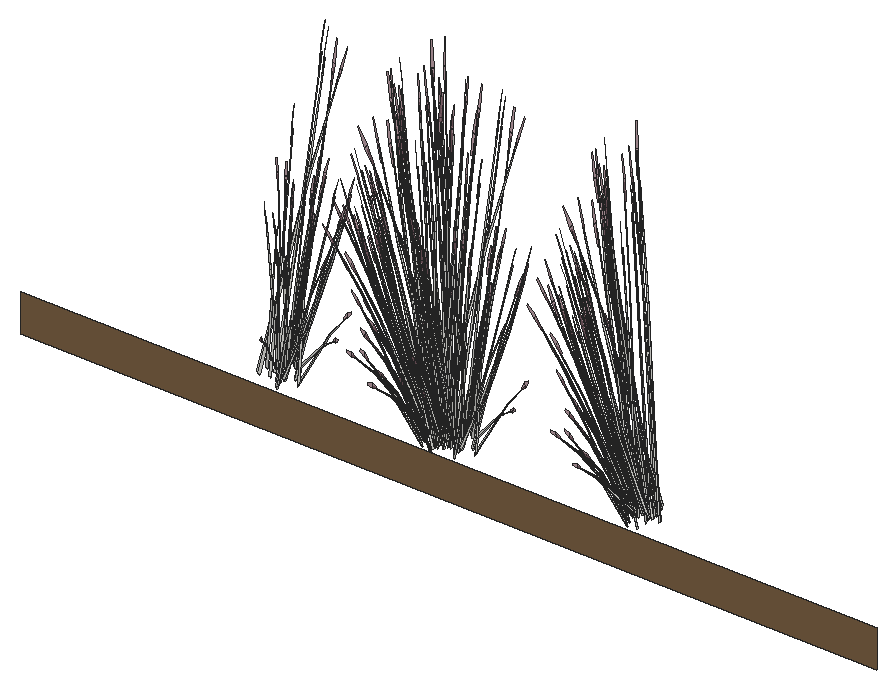
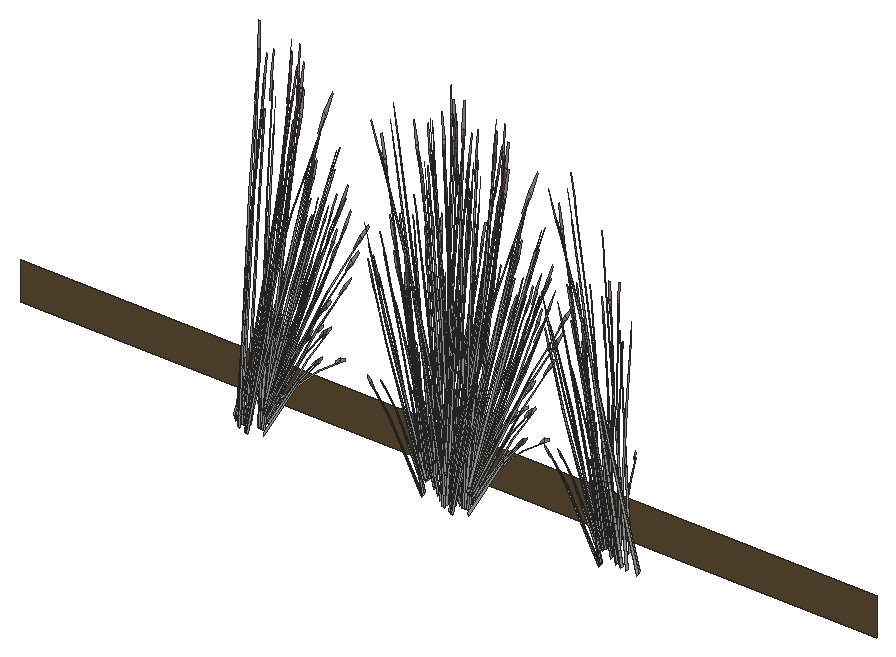
# SketchUp Ruby script. Lengths in inches.
U = 1.inch
M = Sketchup.active_model
def pt(a) = Geom::Point3d.new(a.map { |v| v * U })
def face(e, loops, mat)
  f = e.add_face(loops[0].map { |a| pt(a) })
  loops[1..].each { |l| e.add_face(l.map { |a| pt(a) }).erase! }
  f.material = f.back_material = mat if mat
  f
end
# faces: each face lists its corners as indices into pts; further lists are holes
def faces(e, pts, list, mat = nil) = list.each { |f| face(e, (f[0].is_a?(Array) ? f : [f]).map { |l| l.map { |i| pts[i] } }, mat) }
# xy, xz, yz: faces in a plane at the given z, y or x. An outline is a flat list of corners, or four numbers for a rectangle; further outlines are holes
def ring(l) = l.size == 4 ? [[l[0], l[1]], [l[2], l[1]], [l[2], l[3]], [l[0], l[3]]] : l.each_slice(2).to_a
def flat(e, list, mat, &to3) = list.each { |f| face(e, (f[0].is_a?(Array) ? f : [f]).map { |l| ring(l).map { |u, v| to3.(u, v) } }, mat) }
def xy(e, z, list, mat = nil) = flat(e, list, mat) { |x, y| [x, y, z] }
def xz(e, y, list, mat = nil) = flat(e, list, mat) { |x, z| [x, y, z] }
def yz(e, x, list, mat = nil) = flat(e, list, mat) { |y, z| [x, y, z] }
def lines(e, pts, list) = list.each { |a, b| e.add_line(pt(pts[a]), pt(pts[b])) }
# prism: a flat outline (further loops are holes) pulled along v
def prism(e, loops, v, mat = nil)
  f = face(e, loops, mat); d = Geom::Vector3d.new(v.map { |x| x * U })
  f.pushpull(f.normal.samedirection?(d) ? d.length : -d.length)
end
def box(e, o, s, mat = nil) = prism(e, [[o, [o[0] + s[0], o[1], o[2]], [o[0] + s[0], o[1] + s[1], o[2]], [o[0], o[1] + s[1], o[2]]]], [0, 0, s[2]], mat)
def at(x, y, z, deg = 0) = Geom::Transformation.translation(pt([x, y, z])) * Geom::Transformation.rotation(ORIGIN, Z_AXIS, deg.degrees)
def axes(o, x, y, z) = Geom::Transformation.new([*x, 0, *y, 0, *z, 0, *pt(o).to_a, 1])
def part(name) = M.definitions.add(name)
# library, detail: a bought-in or finely detailed component or shape, given as its bounding box
def library(name, o, s) = part(name).tap { |d| box(d.entities, o, s) }
def detail(e, o, s) = box(e.add_group.entities, o, s)
def put(e, d, t, mat = nil) = e.add_instance(d, t).tap { |i| i.material = mat if mat }
def group(e, t, mat = nil) = e.add_group.tap { |g| g.transformation = t; g.material = mat if mat }.entities
root = M.entities
M.materials.add("LightPink_Translucent").color = [144, 107, 117]
M.materials["LightPink_Translucent"].alpha = 0.75
M.materials.add("Soil_03_1K").color = [122, 96, 67]
c1 = part("blade")
p = [[2.15,0.21,22],[0,0.17,0],[0.09,0.45,0],[2.18,0.31,22],[2.29,0.31,22],[0.38,0.45,0],
  [2.48,0.24,33],[2.49,0.24,33],[2.48,0.22,33]]
faces(c1.entities,p,[[0,1,2,3],[4,5,2,3],[6,3,4,7],[8,0,3,6]])
c2 = part("seeds")
p = [[0.3,-0.1,1.38],[-0.01,-0.03,1.59],[-0.01,-0.03,0.03],[0.14,-0.07,-0.07],[0.29,-0.03,3],[0.15,0.01,3.11]]
faces(c2.entities,p,[[0,1,2,3],[1,0,4,5]],"LightPink_Translucent")
c3 = part("blade with seeds")
put(c3.entities,c1,at(0,0,0))
put(c3.entities,c2,axes([2.4,0.25,30.99],[1.5799,-0.05474,1.17369],[-0.12525,1.92788,0.29478],[-0.07173,-0.02425,1.56792]))
xz(root,2.62,[[45.22,-6,195.77,0.58]],"Soil_03_1K")
put(root,c3,axes([110.6875,10.6,-2.125],[0.17368,0.19618,1.71376],[-0.80256,0.16516,0.13857],[-0.18139,-0.30799,0.73262]))
put(root,c3,axes([146.7,10.6,-2.125],[0.17368,0.19618,1.71376],[-0.80256,0.16516,0.13857],[-0.18139,-0.30799,0.73262]))
put(root,c3,axes([112.01,9.3,-1.28],[-0.11621,-0.08567,1.74944],[-0.77555,0.05431,-0.27667],[-0.12378,-0.20491,0.14031]))
put(root,c3,axes([148.03,9.3,-1.28],[-0.11621,-0.08567,1.74944],[-0.77555,0.05431,-0.27667],[-0.12378,-0.20491,0.14031]))
put(root,c3,axes([113.8125,10.3125,-3.41],[-0.21597,0.12368,1.43002],[-0.64681,-0.21647,-0.30754],[0.1199,-0.26922,0.61141]))
put(root,c3,axes([112.83,10.74,-1.02],[-0.36264,-0.49684,-0.71045],[0.74649,-0.27689,0.08574],[-0.0848,-0.24006,1.00501]))
put(root,c3,axes([148.84,10.74,-1.02],[-0.36264,-0.49684,-0.71045],[0.74649,-0.27689,0.08574],[-0.0848,-0.24006,1.00501]))
put(root,c3,axes([110.47,10.08,-3.41],[-0.04601,0.19989,1.43002],[-0.67263,0.16733,-0.30754],[-0.15723,-0.25836,0.61141]))
put(root,c3,axes([146.48,10.08,-3.41],[-0.04601,0.19989,1.43002],[-0.67263,0.16733,-0.30754],[-0.15723,-0.25836,0.61141]))
put(root,c3,axes([112.2,9.64,-4.51],[-0.12744,0.02202,1.76342],[-0.70477,-0.24781,-0.26939],[0.01183,-0.2067,0.30037]))
put(root,c3,axes([114.34,11.23,-1.02],[0.01977,-0.56521,-0.71045],[0.83252,0.03796,0.08574],[0.08786,-0.23945,1.00501]))
put(root,c3,axes([84.32,10.35,-1.28],[-0.00733,-0.12161,1.74944],[-0.61946,-0.35147,-0.27667],[0.09577,-0.21306,0.14031]))
put(root,c3,axes([115.5,10.35,-1.28],[-0.00733,-0.12161,1.74944],[-0.61946,-0.35147,-0.27667],[0.09577,-0.21306,0.14031]))
put(root,c3,axes([112.9,10.32,-1.47],[0.22906,-0.4699,-0.35414],[0.66828,0.13705,0.4572],[-0.06128,-0.18919,0.87481]))
put(root,c3,axes([82.22,10.94,-2.125],[-0.14147,0.21002,1.71376],[-0.59349,-0.43464,0.13857],[0.26773,-0.27089,0.73262]))
put(root,c3,axes([113.4,10.94,-2.125],[-0.14147,0.21002,1.71376],[-0.59349,-0.43464,0.13857],[0.26773,-0.27089,0.73262]))
put(root,c3,axes([115.33,9.91,-1.29],[-0.07716,0.04667,1.77383],[-0.75601,-0.15746,-0.16761],[-0.02737,-0.20368,0.31391]))
put(root,c3,axes([112.56,10.64,-1.32],[-0.7469,-0.15318,-0.51099],[0.25601,-0.52518,-0.3958],[-0.06849,-0.21144,0.97773]))
put(root,c3,axes([148.57,10.64,-1.32],[-0.7469,-0.15318,-0.51099],[0.25601,-0.52518,-0.3958],[-0.06849,-0.21144,0.97773]))
put(root,c3,axes([113.02,9.33,-3.23],[0.09747,0.35631,1.1486],[-0.54071,-0.19735,0.84392],[0.05818,-0.18244,0.25299]))
put(root,c3,axes([114.17,11.04,-1.32],[-0.54391,-0.41056,-0.51099],[0.57458,-0.35956,-0.3958],[0.08276,-0.2086,0.97773]))
put(root,c3,axes([111.22,9.02,-1.29],[-0.01417,0.07324,1.77383],[-0.6991,0.2658,-0.16761],[-0.20573,-0.13587,0.31391]))
put(root,c3,axes([147.23,9.02,-1.29],[-0.01417,0.07324,1.77383],[-0.6991,0.2658,-0.16761],[-0.20573,-0.13587,0.31391]))
put(root,c3,axes([111.06,10.31,-0.91],[0.84639,-0.15705,0.53763],[0.14689,0.61608,0.4433],[-0.19906,-0.18157,1.11249]))
put(root,c3,axes([147.08,10.31,-0.91],[0.84639,-0.15705,0.53763],[0.14689,0.61608,0.4433],[-0.19906,-0.18157,1.11249]))
put(root,c3,axes([112.98,10.43,-1.27],[0.74868,0.15974,0.48003],[-0.25601,0.52518,0.3958],[-0.04499,-0.20653,0.9933]))
put(root,c3,axes([113.19,10.62,-0.97],[-0.74352,0.28449,-0.1216],[-0.36538,-0.50492,-0.67495],[-0.0981,-0.21277,1.02557]))
put(root,c3,axes([149.21,10.62,-0.97],[-0.74352,0.28449,-0.1216],[-0.36538,-0.50492,-0.67495],[-0.0981,-0.21277,1.02557]))
put(root,c3,axes([114.74,11.26,-0.97],[-0.83505,-0.03027,-0.1216],[0.02282,-0.57322,-0.67495],[0.05801,-0.22077,1.02557]))
put(root,c3,axes([83.5,10.89,-1.47],[0.5141,-0.32171,-0.35414],[0.48666,0.36734,0.4572],[0.07405,-0.18664,0.87481]))
put(root,c3,axes([114.68,10.89,-1.47],[0.5141,-0.32171,-0.35414],[0.48666,0.36734,0.4572],[0.07405,-0.18664,0.87481]))
put(root,c3,axes([110.24,9.76,-3.23],[0.39634,0.21267,1.1486],[-0.57721,0.12784,0.84392],[-0.1235,-0.16344,0.25299]))
put(root,c3,axes([146.25,9.76,-3.23],[0.39634,0.21267,1.1486],[-0.57721,0.12784,0.84392],[-0.1235,-0.16344,0.25299]))
put(root,c3,axes([113.18,10.39,-1.27],[0.55987,-0.20767,0.0643],[0.27403,0.37869,0.50621],[-0.05407,-0.16693,0.77189]))
put(root,c3,axes([111.19,10.88,-1.02],[-0.64788,-0.29534,-0.71045],[0.46044,-0.51755,0.08574],[-0.23473,-0.17635,1.00501]))
put(root,c3,axes([147.21,10.88,-1.02],[-0.64788,-0.29534,-0.71045],[0.46044,-0.51755,0.08574],[-0.23473,-0.17635,1.00501]))
put(root,c3,axes([110.97,10.49,-1.47],[-0.11735,-0.49217,-0.35414],[0.67083,-0.12996,0.4572],[-0.18018,-0.14104,0.87481]))
put(root,c3,axes([146.98,10.49,-1.47],[-0.11735,-0.49217,-0.35414],[0.67083,-0.12996,0.4572],[-0.18018,-0.14104,0.87481]))
put(root,c3,axes([111.26,10.45,-1.27],[0.34533,-0.38816,0.0643],[0.49176,0.22599,0.50621],[-0.15898,-0.12445,0.77189]))
put(root,c3,axes([147.27,10.45,-1.27],[0.34533,-0.38816,0.0643],[0.49176,0.22599,0.50621],[-0.15898,-0.12445,0.77189]))
put(root,c3,axes([109.92,10.4,-4.51],[-0.0736,0.08049,1.76342],[-0.74378,0.17355,-0.26939],[-0.17968,-0.15788,0.30037]))
put(root,c3,axes([145.9375,10.4,-4.51],[-0.0736,0.08049,1.76342],[-0.74378,0.17355,-0.26939],[-0.17968,-0.15788,0.30037]))
put(root,c3,axes([111.15,12.61,-3.9],[-0.31203,-0.62659,-0.69835],[0.89884,-0.22566,-0.18329],[-0.03449,-0.21218,1.54149]))
put(root,c3,axes([147.16,12.61,-3.9],[-0.31203,-0.62659,-0.69835],[0.89884,-0.22566,-0.18329],[-0.03449,-0.21218,1.54149]))
put(root,c3,axes([109.53,11.21,-2.125],[0.28223,0.10528,1.71376],[-0.58406,0.44165,0.13857],[-0.36402,-0.19924,0.73262]))
put(root,c3,axes([145.54,11.21,-2.125],[0.28223,0.10528,1.71376],[-0.58406,0.44165,0.13857],[-0.36402,-0.19924,0.73262]))
put(root,c3,axes([84.15,10.69,-4.51],[-0.11372,-0.04814,1.76342],[-0.29211,-0.53779,-0.26939],[0.19706,-0.14594,0.30037]))
put(root,c3,axes([115.32,10.69,-4.51],[-0.11372,-0.04814,1.76342],[-0.29211,-0.53779,-0.26939],[0.19706,-0.14594,0.30037]))
put(root,c3,axes([112.97,10.82,-0.95],[-0.22906,0.4699,0.35414],[-0.66828,-0.13705,-0.4572],[-0.06128,-0.18919,0.87481]))
put(root,c3,axes([148.98,10.82,-0.95],[-0.22906,0.4699,0.35414],[-0.66828,-0.13705,-0.4572],[-0.06128,-0.18919,0.87481]))
put(root,c3,axes([110.89,10.9,-1.32],[-0.74975,0.14525,-0.51099],[-0.13115,-0.55007,-0.3958],[-0.20138,-0.15763,0.97773]))
put(root,c3,axes([146.9,10.9,-1.32],[-0.74975,0.14525,-0.51099],[-0.13115,-0.55007,-0.3958],[-0.20138,-0.15763,0.97773]))
put(root,c3,axes([83.5,11.01,-1.27],[0.54105,0.41691,0.48003],[-0.57458,0.35956,0.3958],[0.0998,-0.1956,0.9933]))
put(root,c3,axes([114.68,11.01,-1.27],[0.54105,0.41691,0.48003],[-0.57458,0.35956,0.3958],[0.0998,-0.1956,0.9933]))
put(root,c3,axes([111.41,10.41,-0.57],[-0.50709,0.58578,-0.13619],[-0.73436,-0.33748,-0.75594],[-0.25527,-0.1655,1.14864]))
put(root,c3,axes([147.43,10.41,-0.57],[-0.50709,0.58578,-0.13619],[-0.73436,-0.33748,-0.75594],[-0.25527,-0.1655,1.14864]))
put(root,c3,axes([83.7,11.05,-1.27],[0.62439,0.02847,0.0643],[-0.01712,0.42991,0.50621],[0.06534,-0.16468,0.77189]))
put(root,c3,axes([114.88,11.05,-1.27],[0.62439,0.02847,0.0643],[-0.01712,0.42991,0.50621],[0.06534,-0.16468,0.77189]))
put(root,c3,axes([114.41,11.35,-0.95],[-0.5141,0.32171,0.35414],[-0.48666,-0.36734,-0.4572],[0.07405,-0.18664,0.87481]))
put(root,c3,axes([84.14,12.21,-1.02],[0.39688,-0.48213,-0.71045],[0.69548,0.34264,0.08574],[0.23697,-0.17468,1.00501]))
put(root,c3,axes([115.32,12.21,-1.02],[0.39688,-0.48213,-0.71045],[0.69548,0.34264,0.08574],[0.23697,-0.17468,1.00501]))
put(root,c3,axes([111.03,10.81,-3.625],[-0.47504,-0.61229,0],[0.79476,-0.34146,-0.51607],[0.18101,-0.07777,1.63711]))
put(root,c3,axes([84.12,11.99,-1.32],[-0.19519,-0.55794,-0.51099],[0.73919,-0.0976,-0.3958],[0.21183,-0.14986,0.97773]))
put(root,c3,axes([115.3,11.99,-1.32],[-0.19519,-0.55794,-0.51099],[0.73919,-0.0976,-0.3958],[0.21183,-0.14986,0.97773]))
put(root,c3,axes([112.07,10.07,-3.87],[-0.52505,0.35054,-0.03893],[-0.48109,-0.38392,-0.17649],[-0.03387,-0.10878,0.58215]))
put(root,c3,axes([148.08,10.07,-3.87],[-0.52505,0.35054,-0.03893],[-0.48109,-0.38392,-0.17649],[-0.03387,-0.10878,0.58215]))
put(root,c3,axes([109.47,10.24,-1.28],[-0.16348,-0.00431,1.74944],[-0.52047,0.43131,-0.27667],[-0.2777,-0.08813,0.14031]))
put(root,c3,axes([145.48,10.24,-1.28],[-0.16348,-0.00431,1.74944],[-0.52047,0.43131,-0.27667],[-0.2777,-0.08813,0.14031]))
put(root,c3,axes([84.47,12.39,-0.97],[-0.70283,-0.33692,-0.1216],[0.40491,-0.48793,-0.67495],[0.19857,-0.16961,1.02557]))
put(root,c3,axes([115.65,12.39,-0.97],[-0.70283,-0.33692,-0.1216],[0.40491,-0.48793,-0.67495],[0.19857,-0.16961,1.02557]))
put(root,c3,axes([112.74,14.22,-2.67],[0.65659,0.2464,1.51261],[-0.64324,0.53082,0.59816],[-0.28812,-0.31461,1.26806]))
put(root,c3,axes([148.76,14.22,-2.67],[0.65659,0.2464,1.51261],[-0.64324,0.53082,0.59816],[-0.28812,-0.31461,1.26806]))
put(root,c3,axes([111.37,10.89,-0.95],[0.11735,0.49217,0.35414],[-0.67083,0.12996,-0.4572],[-0.18018,-0.14104,0.87481]))
put(root,c3,axes([147.38,10.89,-0.95],[0.11735,0.49217,0.35414],[-0.67083,0.12996,-0.4572],[-0.18018,-0.14104,0.87481]))
put(root,c3,axes([109.3125,12.52,-3.98],[0,-0.61104,-0.49651],[0.85008,0,0],[0,-0.13917,1.57504]))
put(root,c3,axes([145.32,12.52,-3.98],[0,-0.61104,-0.49651],[0.85008,0,0],[0,-0.13917,1.57504]))
put(root,c3,axes([111.67,10.71,-3.98],[0.7111,-0.30552,-0.49651],[0.42504,0.54784,0],[0.16196,-0.06958,1.57504]))
put(root,c3,axes([84.72,11.77,-3.41],[-0.27143,-0.0181,1.43002],[-0.27808,-0.48551,-0.30754],[0.33346,-0.13735,0.61141]))
put(root,c3,axes([115.89,11.77,-3.41],[-0.27143,-0.0181,1.43002],[-0.27808,-0.48551,-0.30754],[0.33346,-0.13735,0.61141]))
put(root,c3,axes([109.35,11.21,-0.91],[0.62747,-0.45094,0.53763],[0.54116,0.47889,0.4433],[-0.29439,-0.08318,1.11249]))
put(root,c3,axes([145.36,11.21,-0.91],[0.62747,-0.45094,0.53763],[0.54116,0.47889,0.4433],[-0.29439,-0.08318,1.11249]))
put(root,c3,axes([86.2,12.24,-1.29],[-0.09924,-0.00464,1.77383],[-0.4121,-0.49725,-0.16761],[0.1655,-0.1635,0.31391]))
put(root,c3,axes([117.38,12.24,-1.29],[-0.09924,-0.00464,1.77383],[-0.4121,-0.49725,-0.16761],[0.1655,-0.1635,0.31391]))
put(root,c3,axes([81.34,11.97,-3.94],[0.51177,-0.45928,-0.62353],[0.63575,0.41646,-0.16365],[0.20507,-0.11457,1.37633]))
put(root,c3,axes([112.52,11.97,-3.94],[0.51177,-0.45928,-0.62353],[0.63575,0.41646,-0.16365],[0.20507,-0.11457,1.37633]))
put(root,c3,axes([85.03,10.875,-3.23],[-0.25308,0.31105,1.1486],[-0.21753,-0.4179,0.84392],[0.20902,-0.10472,0.25299]))
put(root,c3,axes([116.21,10.875,-3.23],[-0.25308,0.31105,1.1486],[-0.21753,-0.4179,0.84392],[0.20902,-0.10472,0.25299]))
put(root,c3,axes([84.67,12.04,-1.47],[0.66138,-0.08733,-0.35414],[0.17464,0.49921,0.4572],[0.18953,-0.13408,0.87481]))
put(root,c3,axes([115.84,12.04,-1.47],[0.66138,-0.08733,-0.35414],[0.17464,0.49921,0.4572],[0.18953,-0.13408,0.87481]))
put(root,c3,axes([109.64,11.21,-1.27],[0.03826,-0.46465,0.0643],[0.57772,0.01274,0.50621],[-0.2213,-0.04862,0.77189]))
put(root,c3,axes([145.65,11.21,-1.27],[0.03826,-0.46465,0.0643],[0.57772,0.01274,0.50621],[-0.2213,-0.04862,0.77189]))
put(root,c3,axes([111.625,12.77,-3.79],[0.36864,-0.55059,-0.44739],[0.76598,0.26498,0.21531],[0,-0.12692,1.43643]))
put(root,c3,axes([109.42,11.36,-1.47],[-0.43232,-0.38257,-0.35414],[0.49364,-0.36215,0.4572],[-0.25081,-0.0551,0.87481]))
put(root,c3,axes([145.43,11.36,-1.47],[-0.43232,-0.38257,-0.35414],[0.49364,-0.36215,0.4572],[-0.25081,-0.0551,0.87481]))
put(root,c3,axes([111.96,12.5,-3.33],[-0.08854,-0.69723,-0.29095],[0.92215,-0.04216,-0.50002],[0.16238,-0.09287,1.59708]))
put(root,c3,axes([109.68,12.54,-3.97],[0.53038,-0.38124,-0.30978],[0.53038,0.38124,0.30978],[0,-0.1228,1.38974]))
put(root,c3,axes([145.6875,12.54,-3.97],[0.53038,-0.38124,-0.30978],[0.53038,0.38124,0.30978],[0,-0.1228,1.38974]))
put(root,c3,axes([109.46,10.71,-3.87],[-0.21918,0.49894,-0.03893],[-0.6746,-0.15348,-0.17649],[-0.10242,-0.08161,0.58215]))
put(root,c3,axes([145.47,10.71,-3.87],[-0.21918,0.49894,-0.03893],[-0.6746,-0.15348,-0.17649],[-0.10242,-0.08161,0.58215]))
put(root,c3,axes([84.13,12.34,-0.95],[-0.66138,0.08733,0.35414],[-0.17464,-0.49921,-0.4572],[0.18953,-0.13408,0.87481]))
put(root,c3,axes([115.3,12.34,-0.95],[-0.66138,0.08733,0.35414],[-0.17464,-0.49921,-0.4572],[0.18953,-0.13408,0.87481]))
put(root,c3,axes([111.53,13.23,-3.33],[-0.85568,-0.29155,-0.29095],[0.41201,-0.61537,-0.50002],[-0.02689,-0.15109,1.59708]))
put(root,c3,axes([147.55,13.23,-3.33],[-0.85568,-0.29155,-0.29095],[0.41201,-0.61537,-0.50002],[-0.02689,-0.15109,1.59708]))
put(root,c3,axes([109.1,12.99,-3.625],[-0.95008,0,0],[0,-0.68292,-0.51607],[0,-0.15554,1.63711]))
put(root,c3,axes([145.11,12.99,-3.625],[-0.95008,0,0],[0,-0.68292,-0.51607],[0,-0.15554,1.63711]))
put(root,c3,axes([109.26,11.76,-3.41],[0.14835,0.17012,1.43002],[-0.34183,0.46242,-0.30754],[-0.351,-0.11053,0.61141]))
put(root,c3,axes([145.27,11.76,-3.41],[0.14835,0.17012,1.43002],[-0.34183,0.46242,-0.30754],[-0.351,-0.11053,0.61141]))
put(root,c3,axes([111.84,10.95,-3.97],[0.70886,0.15119,-0.30978],[-0.17848,0.53243,0.30978],[0.1429,-0.0614,1.38974]))
put(root,c3,axes([109.875,11.61,-1.02],[-0.75952,-0.01471,-0.71045],[0.05101,-0.61953,0.08574],[-0.32177,-0.06538,1.00501]))
put(root,c3,axes([145.89,11.61,-1.02],[-0.75952,-0.01471,-0.71045],[0.05101,-0.61953,0.08574],[-0.32177,-0.06538,1.00501]))
put(root,c3,axes([84.73,12.26,-1.27],[0.52161,0.25698,0.0643],[-0.30368,0.36595,0.50621],[0.16723,-0.11831,0.77189]))
put(root,c3,axes([115.9,12.26,-1.27],[0.52161,0.25698,0.0643],[-0.30368,0.36595,0.50621],[0.16723,-0.11831,0.77189]))
put(root,c3,axes([84.58,12.15,-1.27],[0.18844,0.56237,0.48003],[-0.73919,0.0976,0.3958],[0.21785,-0.13226,0.9933]))
put(root,c3,axes([115.76,12.15,-1.27],[0.18844,0.56237,0.48003],[-0.73919,0.0976,0.3958],[0.21785,-0.13226,0.9933]))
put(root,c3,axes([86.58,12.83,-1.28],[0.10543,-0.09307,1.74944],[-0.13495,-0.57092,-0.27667],[0.26455,-0.10825,0.14031]))
put(root,c3,axes([117.75,12.83,-1.28],[0.10543,-0.09307,1.74944],[-0.13495,-0.57092,-0.27667],[0.26455,-0.10825,0.14031]))
put(root,c3,axes([109.83,12.81,-3.67],[-0.70674,0.51372,0.30756],[-0.70717,-0.50832,-0.36492],[-0.02468,-0.14589,1.64885]))
put(root,c3,axes([145.85,12.81,-3.67],[-0.70674,0.51372,0.30756],[-0.70717,-0.50832,-0.36492],[-0.02468,-0.14589,1.64885]))
put(root,c3,axes([108.84,10.6,-1.29],[0.05633,0.06098,1.77383],[-0.27155,0.54815,-0.16761],[-0.27501,0.00397,0.31391]))
put(root,c3,axes([144.86,10.6,-1.29],[0.05633,0.06098,1.77383],[-0.27155,0.54815,-0.16761],[-0.27501,0.00397,0.31391]))
put(root,c3,axes([112.08,13.04,-3.57],[0.8561,0.29616,0.24065],[-0.41201,0.61537,0.50002],[0,-0.14185,1.60543]))
put(root,c3,axes([111.75,13.875,-3.5625],[0.20138,-0.72405,-0.23429],[0.95485,0.12621,0.51271],[-0.16685,-0.09999,1.5644]))
put(root,c3,axes([147.76,13.875,-3.5625],[0.20138,-0.72405,-0.23429],[0.95485,0.12621,0.51271],[-0.16685,-0.09999,1.5644]))
put(root,c3,axes([109.62,11.74,-1.32],[-0.55171,0.40476,-0.51099],[-0.48318,-0.42758,-0.3958],[-0.28031,-0.06159,0.97773]))
put(root,c3,axes([145.63,11.74,-1.32],[-0.55171,0.40476,-0.51099],[-0.48318,-0.42758,-0.3958],[-0.28031,-0.06159,0.97773]))
put(root,c3,axes([110.03,11.56,-0.95],[0.43232,0.38257,0.35414],[-0.49364,0.36215,-0.4572],[-0.25081,-0.0551,0.87481]))
put(root,c3,axes([146.04,11.56,-0.95],[0.43232,0.38257,0.35414],[-0.49364,0.36215,-0.4572],[-0.25081,-0.0551,0.87481]))
put(root,c3,axes([108.38,12.28,-3.23],[0.48508,-0.04372,1.1486],[-0.3077,0.38525,0.84392],[-0.23971,-0.05779,0.25299]))
put(root,c3,axes([144.39,12.28,-3.23],[0.48508,-0.04372,1.1486],[-0.3077,0.38525,0.84392],[-0.23971,-0.05779,0.25299]))
put(root,c3,axes([111.81,12.63,-3.28],[-0.82508,0.03772,0.44739],[-0.07462,-0.62614,-0.21531],[0.14771,-0.06346,1.43643]))
put(root,c3,axes([109.91,11.32,-0.97],[-0.04068,0.62141,-0.1216],[-0.77029,-0.01698,-0.67495],[-0.29667,-0.04317,1.02557]))
put(root,c3,axes([145.92,11.32,-0.97],[-0.04068,0.62141,-0.1216],[-0.77029,-0.01698,-0.67495],[-0.29667,-0.04317,1.02557]))
put(root,c3,axes([109.68,13.09,-3.52],[0,0.61104,0.49651],[-0.85008,0,0],[0,-0.13917,1.57504]))
put(root,c3,axes([145.6875,13.09,-3.52],[0,0.61104,0.49651],[-0.85008,0,0],[0,-0.13917,1.57504]))
put(root,c3,axes([84.5,13.7,-0.97],[-0.38229,-0.5533,-0.1216],[0.6785,-0.2719,-0.67495],[0.28593,-0.073,1.02557]))
put(root,c3,axes([115.68,13.7,-0.97],[-0.38229,-0.5533,-0.1216],[0.6785,-0.2719,-0.67495],[0.28593,-0.073,1.02557]))
put(root,c3,axes([84.47,13.22,-1.32],[0.20584,-0.55581,-0.51099],[0.70573,0.19051,-0.3958],[0.28414,-0.05097,0.97773]))
put(root,c3,axes([115.64,13.22,-1.32],[0.20584,-0.55581,-0.51099],[0.70573,0.19051,-0.3958],[0.28414,-0.05097,0.97773]))
put(root,c3,axes([83.35,10.96,-3.625],[0.47504,-0.61229,0],[0.79476,0.34146,-0.51607],[0.18101,0.07777,1.63711]))
put(root,c3,axes([114.53,10.96,-3.625],[0.47504,-0.61229,0],[0.79476,0.34146,-0.51607],[0.18101,0.07777,1.63711]))
put(root,c3,axes([108.93,12.17,-2.125],[0.31515,-0.01384,1.71376],[-0.20907,0.5998,0.13857],[-0.44912,-0.0371,0.73262]))
put(root,c3,axes([144.94,12.17,-2.125],[0.31515,-0.01384,1.71376],[-0.20907,0.5998,0.13857],[-0.44912,-0.0371,0.73262]))
put(root,c3,axes([111.68,13.58,-3.79],[-0.45644,-0.51287,-0.44739],[0.69137,-0.36116,0.21531],[-0.14771,-0.06346,1.43643]))
put(root,c3,axes([147.7,13.58,-3.79],[-0.45644,-0.51287,-0.44739],[0.69137,-0.36116,0.21531],[-0.14771,-0.06346,1.43643]))
put(root,c3,axes([111.78,12.86,-3.64],[0.33034,0.68327,0.45755],[-0.94388,0.2376,0.17955],[0.01154,-0.12555,1.58856]))
put(root,c3,axes([85.22,13.38,-4.02],[-0.48937,0.07333,1.41583],[-0.07789,-0.58369,0.08104],[0.34275,-0.08835,0.80566]))
put(root,c3,axes([116.4,13.38,-4.02],[-0.48937,0.07333,1.41583],[-0.07789,-0.58369,0.08104],[0.34275,-0.08835,0.80566]))
put(root,c3,axes([86.11,12.86,-3.74],[-0.47106,-0.39072,-0.06488],[0.51591,-0.35801,-0.29416],[0.14618,-0.02521,0.97024]))
put(root,c3,axes([117.29,12.86,-3.74],[-0.47106,-0.39072,-0.06488],[0.51591,-0.35801,-0.29416],[0.14618,-0.02521,0.97024]))
put(root,c3,axes([111.61,13.4,-3.28],[-0.36864,0.55059,0.44739],[-0.76598,-0.26498,-0.21531],[0,-0.12692,1.43643]))
put(root,c3,axes([147.625,13.4,-3.28],[-0.36864,0.55059,0.44739],[-0.76598,-0.26498,-0.21531],[0,-0.12692,1.43643]))
put(root,c3,axes([112.97,12.92,-3.79],[0,-0.70701,0],[0.95008,0,0],[0,0,1.79456]))
put(root,c3,axes([114.12,11.28,-3.52],[-0.7111,-0.30552,0.49651],[0.42504,-0.54784,0],[0.16196,0.06958,1.57504]))
put(root,c3,axes([84.33,13.43,-1.02],[0.66765,-0.26986,-0.71045],[0.37208,0.55551,0.08574],[0.32259,-0.0631,1.00501]))
put(root,c3,axes([115.51,13.43,-1.02],[0.66765,-0.26986,-0.71045],[0.37208,0.55551,0.08574],[0.32259,-0.0631,1.00501]))
put(root,c3,axes([111.27,13.78,-3.94],[-0.79037,-0.10018,-0.62353],[0.16679,-0.61794,-0.16365],[-0.23587,-0.07488,1.37633]))
put(root,c3,axes([147.29,13.78,-3.94],[-0.79037,-0.10018,-0.62353],[0.16679,-0.61794,-0.16365],[-0.23587,-0.07488,1.37633]))
put(root,c3,axes([112.51,12.47,-3.64],[-0.62999,0.55453,0.45755],[-0.74845,-0.4895,0.17955],[0.15188,-0.05534,1.58856]))
put(root,c3,axes([113.2,13.46,-3.7],[-0.70674,-0.52593,-0.06131],[0.70717,-0.52625,0],[-0.02468,-0.01837,1.75571]))
put(root,c3,axes([149.22,13.46,-3.7],[-0.70674,-0.52593,-0.06131],[0.70717,-0.52625,0],[-0.02468,-0.01837,1.75571]))
put(root,c3,axes([111.42,11.56,-3.53],[-0.21949,0.60727,0.17642],[-0.8032,-0.17185,0.35086],[0.13875,-0.00296,1.60407]))
put(root,c3,axes([84.23,13.53,-0.95],[-0.63144,-0.17046,0.35414],[0.18417,-0.49731,-0.4572],[0.25423,-0.0456,0.87481]))
put(root,c3,axes([115.41,13.53,-0.95],[-0.63144,-0.17046,0.35414],[0.18417,-0.49731,-0.4572],[0.25423,-0.0456,0.87481]))
put(root,c3,axes([108.8,12.625,-1.27],[0.21466,-0.55714,0.48003],[0.70573,0.19051,0.3958],[-0.27753,0.03348,0.9933]))
put(root,c3,axes([144.8125,12.625,-1.27],[0.21466,-0.55714,0.48003],[0.70573,0.19051,0.3958],[-0.27753,0.03348,0.9933]))
put(root,c3,axes([79.91,12.05,-4.41],[-0.74787,0.24464,1.28929],[-0.23804,-0.70192,0.50096],[0.45924,0.01168,1.46642]))
put(root,c3,axes([111.09,12.05,-4.41],[-0.74787,0.24464,1.28929],[-0.23804,-0.70192,0.50096],[0.45924,0.01168,1.46642]))
put(root,c3,axes([113.1,12.23,-3.38],[0.14658,-0.54532,0.1448],[0.71613,0.09466,-0.41347],[0.13033,0.05599,1.26744]))
put(root,c3,axes([108.75,12.48,-1.27],[-0.27906,-0.41663,0.0643],[0.50888,-0.20393,0.50621],[-0.22432,0.04024,0.77189]))
put(root,c3,axes([144.76,12.48,-1.27],[-0.27906,-0.41663,0.0643],[0.50888,-0.20393,0.50621],[-0.22432,0.04024,0.77189]))
put(root,c3,axes([111.86,13.53,-3.64],[0.96033,0.12874,0.45755],[-0.19544,0.7271,0.17955],[-0.14034,-0.07021,1.58856]))
put(root,c3,axes([147.875,13.53,-3.64],[0.96033,0.12874,0.45755],[-0.19544,0.7271,0.17955],[-0.14034,-0.07021,1.58856]))
put(root,c3,axes([85.75,13,-4.51],[-0.03971,-0.09277,1.76342],[0.27541,-0.54264,-0.26939],[0.27782,-0.00781,0.30037]))
put(root,c3,axes([116.93,13,-4.51],[-0.03971,-0.09277,1.76342],[0.27541,-0.54264,-0.26939],[0.27782,-0.00781,0.30037]))
put(root,c3,axes([108.73,12.91,-4.51],[0.01927,0.0963,1.76342],[-0.38846,0.5029,-0.26939],[-0.27592,-0.02535,0.30037]))
put(root,c3,axes([144.75,12.91,-4.51],[0.01927,0.0963,1.76342],[-0.38846,0.5029,-0.26939],[-0.27592,-0.02535,0.30037]))
put(root,c3,axes([112.79,12.375,-3.28],[-0.45644,-0.51287,0.44739],[0.69137,-0.36116,-0.21531],[0.14771,0.06346,1.43643]))
put(root,c3,axes([110.43,14.72,-3.97],[-0.17848,-0.53243,-0.30978],[0.70886,-0.15119,0.30978],[-0.1429,-0.0614,1.38974]))
put(root,c3,axes([146.45,14.72,-3.97],[-0.17848,-0.53243,-0.30978],[0.70886,-0.15119,0.30978],[-0.1429,-0.0614,1.38974]))
put(root,c3,axes([111.34,14.6875,-3.53],[0.81646,-0.16218,0.17642],[0.20161,0.60355,0.35086],[-0.07282,-0.08794,1.60407]))
put(root,c3,axes([147.36,14.6875,-3.53],[0.81646,-0.16218,0.17642],[0.20161,0.60355,0.35086],[-0.07282,-0.08794,1.60407]))
put(root,c3,axes([81.85,12.41,-3.33],[0.76714,-0.40567,-0.29095],[0.51013,0.57321,-0.50002],[0.18927,0.05821,1.59708]))
put(root,c3,axes([113.03,12.41,-3.33],[0.76714,-0.40567,-0.29095],[0.51013,0.57321,-0.50002],[0.18927,0.05821,1.59708]))
put(root,c3,axes([84.9,13.48,-1.47],[0.63144,0.17046,-0.35414],[-0.18417,0.49731,0.4572],[0.25423,-0.0456,0.87481]))
put(root,c3,axes([116.08,13.48,-1.47],[0.63144,0.17046,-0.35414],[-0.18417,0.49731,0.4572],[0.25423,-0.0456,0.87481]))
put(root,c3,axes([110.24,14.95,-3.98],[-0.7111,-0.30552,-0.49651],[0.42504,-0.54784,0],[-0.16196,-0.06958,1.57504]))
put(root,c3,axes([146.25,14.95,-3.98],[-0.7111,-0.30552,-0.49651],[0.42504,-0.54784,0],[-0.16196,-0.06958,1.57504]))
put(root,c3,axes([83.78,11.33,-3.98],[0.7111,0.30552,-0.49651],[-0.42504,0.54784,0],[0.16196,0.06958,1.57504]))
put(root,c3,axes([114.96,11.33,-3.98],[0.7111,0.30552,-0.49651],[-0.42504,0.54784,0],[0.16196,0.06958,1.57504]))
put(root,c3,axes([108.65,12.6875,-1.47],[-0.63144,-0.17046,-0.35414],[0.18417,-0.49731,0.4572],[-0.25423,0.0456,0.87481]))
put(root,c3,axes([144.67,12.6875,-1.47],[-0.63144,-0.17046,-0.35414],[0.18417,-0.49731,0.4572],[-0.25423,0.0456,0.87481]))
